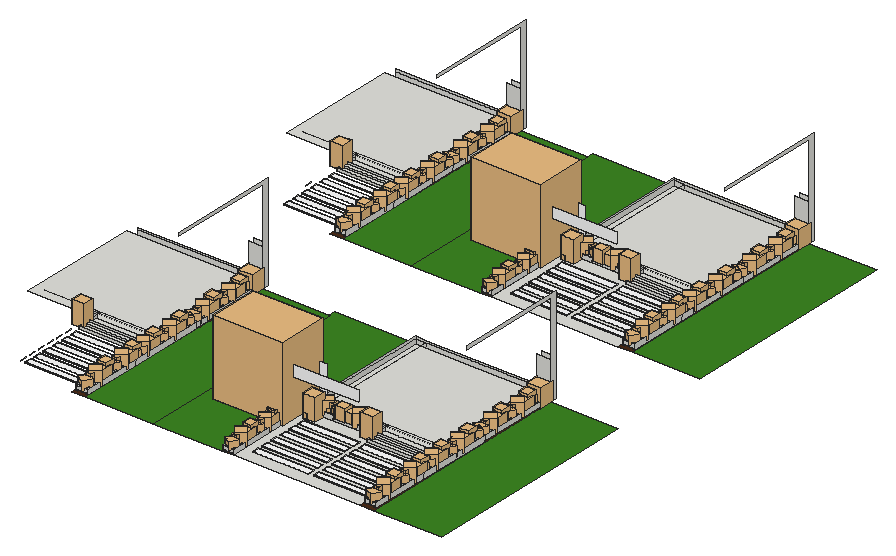
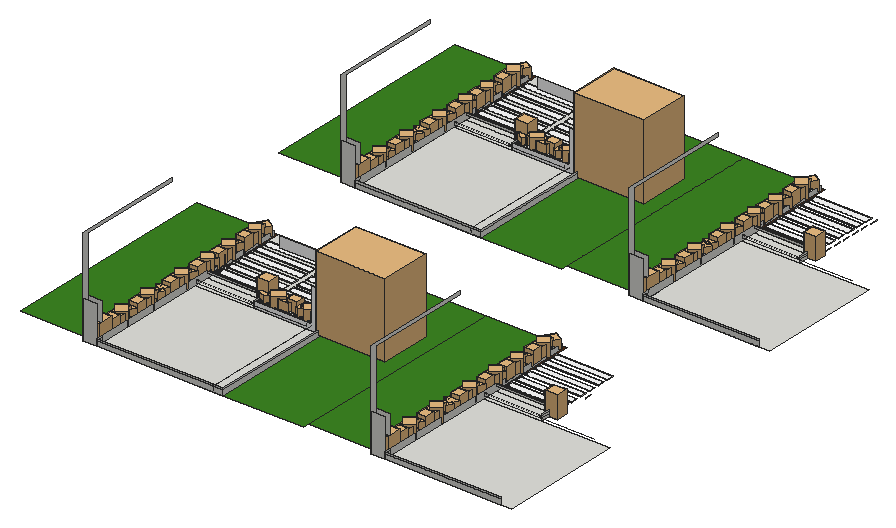
# SketchUp Ruby script. Lengths in inches.
U = 1.inch
M = Sketchup.active_model
def pt(a) = Geom::Point3d.new(a.map { |v| v * U })
def face(e, loops, mat)
  f = e.add_face(loops[0].map { |a| pt(a) })
  loops[1..].each { |l| e.add_face(l.map { |a| pt(a) }).erase! }
  f.material = f.back_material = mat if mat
  f
end
# faces: each face lists its corners as indices into pts; further lists are holes
def faces(e, pts, list, mat = nil) = list.each { |f| face(e, (f[0].is_a?(Array) ? f : [f]).map { |l| l.map { |i| pts[i] } }, mat) }
# xy, xz, yz: faces in a plane at the given z, y or x. An outline is a flat list of corners, or four numbers for a rectangle; further outlines are holes
def ring(l) = l.size == 4 ? [[l[0], l[1]], [l[2], l[1]], [l[2], l[3]], [l[0], l[3]]] : l.each_slice(2).to_a
def flat(e, list, mat, &to3) = list.each { |f| face(e, (f[0].is_a?(Array) ? f : [f]).map { |l| ring(l).map { |u, v| to3.(u, v) } }, mat) }
def xy(e, z, list, mat = nil) = flat(e, list, mat) { |x, y| [x, y, z] }
def xz(e, y, list, mat = nil) = flat(e, list, mat) { |x, z| [x, y, z] }
def yz(e, x, list, mat = nil) = flat(e, list, mat) { |y, z| [x, y, z] }
def lines(e, pts, list) = list.each { |a, b| e.add_line(pt(pts[a]), pt(pts[b])) }
# prism: a flat outline (further loops are holes) pulled along v
def prism(e, loops, v, mat = nil)
  f = face(e, loops, mat); d = Geom::Vector3d.new(v.map { |x| x * U })
  f.pushpull(f.normal.samedirection?(d) ? d.length : -d.length)
end
def box(e, o, s, mat = nil) = prism(e, [[o, [o[0] + s[0], o[1], o[2]], [o[0] + s[0], o[1] + s[1], o[2]], [o[0], o[1] + s[1], o[2]]]], [0, 0, s[2]], mat)
def at(x, y, z, deg = 0) = Geom::Transformation.translation(pt([x, y, z])) * Geom::Transformation.rotation(ORIGIN, Z_AXIS, deg.degrees)
def axes(o, x, y, z) = Geom::Transformation.new([*x, 0, *y, 0, *z, 0, *pt(o).to_a, 1])
def part(name) = M.definitions.add(name)
# library, detail: a bought-in or finely detailed component or shape, given as its bounding box
def library(name, o, s) = part(name).tap { |d| box(d.entities, o, s) }
def detail(e, o, s) = box(e.add_group.entities, o, s)
def put(e, d, t, mat = nil) = e.add_instance(d, t).tap { |i| i.material = mat if mat }
def group(e, t, mat = nil) = e.add_group.tap { |g| g.transformation = t; g.material = mat if mat }.entities
root = M.entities
M.materials.add("Material__1").color = [95, 70, 46]
M.materials.add("[Carrera Marble]").color = [255, 255, 255]
M.materials.add("[Color M00]").color = [255, 255, 255]
M.materials.add("[Color M04]").color = [60, 133, 34]
M.materials.add("[Wood Veneer 01]").color = [76, 44, 23]
c1 = library("plant1",[-367.84,-375.82,-125.45],[750.59,696.16,1346.74])
c2 = part("skp4FF")
put(c2.entities,c1,at(0,0,0))
c3 = library("Areca palm plant",[0,0,0],[49.1,36.6,54.46])
c4 = library("Group\#14",[-84.69,-90.07,-0.36],[176.51,175.13,171.4])
c5 = library("Group20\#1",[-20.81,-17.08,3.79],[39.86,39.43,37.51])
c6 = library("Group\#130",[-7.34,-1.2,0],[38.67,35.81,49.04])
c7 = library("Group38\#2",[14.01,28.44,-23.43],[18.58,18.32,38.89])
c8 = part("Group\#15")
xy(c8.entities,0,[[0,0,6,234.8],[30,0,36,234.8]])
xy(c8.entities,3,[[6,0,30,234.8]])
xy(c8.entities,7,[[6,5,30,229.8]],"Material__1")
xy(c8.entities,15,[[[0,0,36,234.8],[6,5,30,229.8]]])
xz(c8.entities,0,[[0,0,6,0,6,3,30,3,30,0,36,0,36,15,0,15]])
xz(c8.entities,5,[[6,7,30,15]])
xz(c8.entities,229.8,[[6,7,30,15]])
xz(c8.entities,234.8,[[0,0,0,15,36,15,36,0,30,0,30,3,6,3,6,0]])
yz(c8.entities,0,[[0,0,234.8,15]])
yz(c8.entities,6,[[0,0,234.8,3],[5,7,229.8,15]])
yz(c8.entities,30,[[0,0,234.8,3],[5,7,229.8,15]])
yz(c8.entities,36,[[0,0,234.8,15]])
c9 = part("Group\#17")
put(c9.entities,c3,axes([-6.2,56.6,6.08],[0.45017,-0.56191,0],[0.66137,0.52986,0],[0,0,0.72]))
put(c9.entities,c3,axes([-6.2,158.41,6.08],[0.45017,-0.56191,0],[0.66137,0.52986,0],[0,0,0.72]))
put(c9.entities,c4,axes([14.93,44.05,6.05],[-0.04961,-0.08593,0],[0.08593,-0.04961,0],[0,0,0.10522]))
put(c9.entities,c4,axes([14.93,71.3,6.05],[-0.04961,-0.08593,0],[0.08593,-0.04961,0],[0,0,0.10522]))
put(c9.entities,c5,axes([18.97,79.98,4.77],[0,0.85,0],[-0.85,0,0],[0,0,0.85]))
put(c9.entities,c4,axes([14.93,145.87,6.05],[-0.04961,-0.08593,0],[0.08593,-0.04961,0],[0,0,0.10522]))
put(c9.entities,c4,axes([17.19,15.79,6.07],[-0.08133,-0.14087,0],[0.14087,-0.08133,0],[0,0,0.1725]))
put(c9.entities,c4,axes([17.19,223.04,6.07],[-0.08133,-0.14087,0],[0.14087,-0.08133,0],[0,0,0.1725]))
put(c9.entities,c4,axes([17.19,121.23,6.07],[-0.08133,-0.14087,0],[0.14087,-0.08133,0],[0,0,0.1725]))
put(c9.entities,c6,axes([24.9375,191.72,8],[0,0.79,0],[-0.79,0,0],[0,0,0.79]))
put(c9.entities,c6,axes([24.9375,89.91,8],[0,0.79,0],[-0.79,0,0],[0,0,0.79]))
put(c9.entities,c4,axes([14.93,91.37,6.05],[-0.04961,-0.08593,0],[0.08593,-0.04961,0],[0,0,0.10522]))
put(c9.entities,c5,axes([18.97,181.79,4.77],[0,0.85,0],[-0.85,0,0],[0,0,0.85]))
put(c9.entities,c7,axes([-4.1,-1.15,28.17],[0.8848,0,0],[0,0.94674,0],[0,0,0.85826]))
put(c9.entities,c7,axes([-4.1,100.66,28.17],[0.8848,0,0],[0,0.94674,0],[0,0,0.85826]))
put(c9.entities,c8,at(0,0,0))
put(c9.entities,c4,axes([14.93,173.12,6.05],[-0.04961,-0.08593,0],[0.08593,-0.04961,0],[0,0,0.10522]))
put(c9.entities,c4,axes([14.93,193.18,6.05],[-0.04961,-0.08593,0],[0.08593,-0.04961,0],[0,0,0.10522]))
c10 = library("plant (1)",[-35.72,-28.42,0],[66.31,67.39,84.38])
c11 = library("Group\#18",[0,0,0],[68.35,49.34,73.02])
c12 = library("Plant",[0,0,0],[12.59,12.59,14.16])
c13 = part("Group\#16")
put(c13.entities,c3,axes([-6.2,158.41,6.08],[0.45017,-0.56191,0],[0.66137,0.52986,0],[0,0,0.72]))
put(c13.entities,c3,axes([-6.2,56.6,6.08],[0.45017,-0.56191,0],[0.66137,0.52986,0],[0,0,0.72]))
put(c13.entities,c4,axes([14.93,91.37,6.05],[-0.04961,-0.08593,0],[0.08593,-0.04961,0],[0,0,0.10522]))
put(c13.entities,c4,axes([14.93,145.87,6.05],[-0.04961,-0.08593,0],[0.08593,-0.04961,0],[0,0,0.10522]))
put(c13.entities,c4,axes([17.19,223.04,6.07],[-0.08133,-0.14087,0],[0.14087,-0.08133,0],[0,0,0.1725]))
put(c13.entities,c8,at(0,0,0))
put(c13.entities,c4,axes([14.93,193.18,6.05],[-0.04961,-0.08593,0],[0.08593,-0.04961,0],[0,0,0.10522]))
put(c13.entities,c4,axes([17.19,15.79,6.07],[-0.08133,-0.14087,0],[0.14087,-0.08133,0],[0,0,0.1725]))
put(c13.entities,c5,axes([18.97,181.79,4.77],[0,0.85,0],[-0.85,0,0],[0,0,0.85]))
put(c13.entities,c5,axes([18.97,79.98,4.77],[0,0.85,0],[-0.85,0,0],[0,0,0.85]))
put(c13.entities,c7,axes([-4.1,-1.15,28.17],[0.8848,0,0],[0,0.94674,0],[0,0,0.85826]))
put(c13.entities,c7,axes([-4.1,100.66,28.17],[0.8848,0,0],[0,0.94674,0],[0,0,0.85826]))
put(c13.entities,c6,axes([24.9375,89.91,8],[0,0.79,0],[-0.79,0,0],[0,0,0.79]))
put(c13.entities,c4,axes([14.93,173.12,6.05],[-0.04961,-0.08593,0],[0.08593,-0.04961,0],[0,0,0.10522]))
put(c13.entities,c4,axes([14.93,44.05,6.05],[-0.04961,-0.08593,0],[0.08593,-0.04961,0],[0,0,0.10522]))
put(c13.entities,c4,axes([14.93,71.3,6.05],[-0.04961,-0.08593,0],[0.08593,-0.04961,0],[0,0,0.10522]))
put(c13.entities,c6,axes([24.9375,191.72,8],[0,0.79,0],[-0.79,0,0],[0,0,0.79]))
put(c13.entities,c4,axes([17.19,121.23,6.07],[-0.08133,-0.14087,0],[0.14087,-0.08133,0],[0,0,0.1725]))
xy(root,-14.85,[[[2957.51,315.5,3349.13,315.5,3349.13,568.0625,3169.48,568.0625,3169.48,636.6875,2957.51,636.6875,2957.51,593.125,2930.51,593.125,2930.51,586.4375,2957.51,586.4375],[3171.73,497.23,3345.23,518.73],[2983.23,497.23,3156.73,518.73],[3171.73,532.29,3345.23,553.79],[3171.73,462.17,3345.23,483.67],[3171.73,427.11,3345.23,448.61],[3171.73,392.04,3345.23,413.54],[3171.73,356.98,3345.23,378.48],[2983.23,532.29,3156.73,553.79],[2983.23,462.17,3156.73,483.67],[2983.23,427.11,3156.73,448.61],[2983.23,392.04,3156.73,413.54],[2983.23,356.98,3156.73,378.48]],[2930.51,536.1875,2957.51,586.4375],[2276.89,568.0625,2456.54,590.5625],[3169.48,568.0625,3349.13,590.5625],[2276.89,590.5625,2456.54,636.6875],
  [3169.48,590.5625,3349.13,636.6875],[2064.92,636.6875,2456.54,1019],[2957.51,636.6875,3349.13,1019],[2456.54,999.35,2500.29,1019],[3349.13,999.35,3392.88,1019],
  [[2957.51,1314.85,3349.13,1314.85,3349.13,1567.42,3169.48,1567.42,3169.48,1636.04,2957.51,1636.04,2957.51,1592.48,2930.51,1592.48,2930.51,1585.79,2957.51,1585.79],[3171.73,1531.65,3345.23,1553.15],[3171.73,1496.59,3345.23,1518.09],[3171.73,1461.52,3345.23,1483.02],[3171.73,1426.46,3345.23,1447.96],[3171.73,1391.4,3345.23,1412.9],[3171.73,1356.34,3345.23,1377.84],[2983.23,1531.65,3156.73,1553.15],[2983.23,1496.59,3156.73,1518.09],[2983.23,1461.52,3156.73,1483.02],[2983.23,1426.46,3156.73,1447.96],[2983.23,1391.4,3156.73,1412.9],[2983.23,1356.34,3156.73,1377.84]],[2930.51,1535.54,2957.51,1585.79],[2276.89,1567.42,2456.54,1589.92],[3169.48,1567.42,3349.13,1589.92],[2276.89,1589.92,2456.54,1636.04],
  [3169.48,1589.92,3349.13,1636.04],[2064.92,1636.04,2456.54,2018.36],[2957.51,1636.04,3349.13,2018.36],[2456.54,1998.71,2500.29,2018.36],[3349.13,1998.71,3392.88,2018.36]])
xy(root,-14.85,[[2500.29,315.5,2708.22,999.35],[[2708.22,315.5,2930.51,315.5,2930.51,593.125,2957.51,593.125,2957.51,1019,2708.22,1019],[2851.78,562.6,2854.94,565.76,2854.94,562.6]],[3392.88,315.5,3600.8125,999.35],[2851.78,562.6,2854.94,562.6,2854.94,565.76],[2500.29,1314.85,2708.22,1998.71],
  [[2708.22,1314.85,2930.51,1314.85,2930.51,1592.48,2957.51,1592.48,2957.51,2018.36,2708.22,2018.36],[2851.78,1561.96,2854.94,1565.12,2854.94,1561.96]],[3392.88,1314.85,3600.8125,1998.71],[2851.78,1561.96,2854.94,1561.96,2854.94,1565.12]],"[Color M04]")
xy(root,-14.85,[[2456.54,315.5,2500.29,999.35],[2930.51,315.5,2957.51,536.1875],[3349.13,315.5,3392.88,999.35],[2456.54,1314.85,2500.29,1998.71],[2930.51,1314.85,2957.51,1535.54],
  [3349.13,1314.85,3392.88,1998.71]],"[Wood Veneer 01]")
xy(root,-13.54,[[2279.14,356.98,2452.64,378.48],[2983.23,356.98,3156.73,378.48],[3171.73,356.98,3345.23,378.48],[2279.14,392.04,2452.64,413.54],[2983.23,392.04,3156.73,413.54],
  [3171.73,392.04,3345.23,413.54],[2279.14,427.11,2452.64,448.61],[2983.23,427.11,3156.73,448.61],[3171.73,427.11,3345.23,448.61],[2279.14,462.17,2452.64,483.67],
  [2983.23,462.17,3156.73,483.67],[3171.73,462.17,3345.23,483.67],[2279.14,497.23,2452.64,518.73],[2983.23,497.23,3156.73,518.73],[3171.73,497.23,3345.23,518.73],
  [2279.14,532.29,2452.64,553.79],[2983.23,532.29,3156.73,553.79],[3171.73,532.29,3345.23,553.79],[2279.14,1356.34,2452.64,1377.84],[2983.23,1356.34,3156.73,1377.84],
  [3171.73,1356.34,3345.23,1377.84],[2279.14,1391.4,2452.64,1412.9],[2983.23,1391.4,3156.73,1412.9],[3171.73,1391.4,3345.23,1412.9],[2279.14,1426.46,2452.64,1447.96],
  [2983.23,1426.46,3156.73,1447.96],[3171.73,1426.46,3345.23,1447.96],[2279.14,1461.52,2452.64,1483.02],[2983.23,1461.52,3156.73,1483.02],[3171.73,1461.52,3345.23,1483.02],
  [2279.14,1496.59,2452.64,1518.09],[2983.23,1496.59,3156.73,1518.09],[3171.73,1496.59,3345.23,1518.09],[2279.14,1531.65,2452.64,1553.15],[2983.23,1531.65,3156.73,1553.15],
  [3171.73,1531.65,3345.23,1553.15]],"[Carrera Marble]")
xy(root,-6.43,[[2276.89,568.0625,2456.54,579.9375],[3169.48,568.0625,3349.13,579.9375],[2276.89,1567.42,2456.54,1579.29],[3169.48,1567.42,3349.13,1579.29]])
xy(root,-0.05,[[2276.89,579.9375,2456.54,590.5625],[3169.48,579.9375,3349.13,590.5625],[2276.89,1579.29,2456.54,1589.92],[3169.48,1579.29,3349.13,1589.92]])
xz(root,356.98,[[2279.14,-14.85,2452.64,-13.54],[2983.23,-14.85,3156.73,-13.54],[3171.73,-14.85,3345.23,-13.54]])
xz(root,378.48,[[2279.14,-14.85,2452.64,-13.54],[2983.23,-14.85,3156.73,-13.54],[3171.73,-14.85,3345.23,-13.54]])
xz(root,392.04,[[2279.14,-14.85,2452.64,-13.54],[2983.23,-14.85,3156.73,-13.54],[3171.73,-14.85,3345.23,-13.54]])
xz(root,413.54,[[2279.14,-14.85,2452.64,-13.54],[2983.23,-14.85,3156.73,-13.54],[3171.73,-14.85,3345.23,-13.54]])
xz(root,427.11,[[2279.14,-14.85,2452.64,-13.54],[2983.23,-14.85,3156.73,-13.54],[3171.73,-14.85,3345.23,-13.54]])
xz(root,448.61,[[2279.14,-14.85,2452.64,-13.54],[2983.23,-14.85,3156.73,-13.54],[3171.73,-14.85,3345.23,-13.54]])
xz(root,462.17,[[2279.14,-14.85,2452.64,-13.54],[2983.23,-14.85,3156.73,-13.54],[3171.73,-14.85,3345.23,-13.54]])
xz(root,483.67,[[2279.14,-14.85,2452.64,-13.54],[2983.23,-14.85,3156.73,-13.54],[3171.73,-14.85,3345.23,-13.54]])
xz(root,497.23,[[2279.14,-14.85,2452.64,-13.54],[2983.23,-14.85,3156.73,-13.54],[3171.73,-14.85,3345.23,-13.54]])
xz(root,518.73,[[2279.14,-14.85,2452.64,-13.54],[2983.23,-14.85,3156.73,-13.54],[3171.73,-14.85,3345.23,-13.54]])
xz(root,532.29,[[2279.14,-14.85,2452.64,-13.54],[2983.23,-14.85,3156.73,-13.54],[3171.73,-14.85,3345.23,-13.54]])
xz(root,536.1875,[[2930.51,-14.85,2957.51,-14.85,2957.51,109.625,3169.48,109.625,3169.48,142.875,2930.51,142.875]],"[Color M00]")
xz(root,553.79,[[2279.14,-14.85,2452.64,-13.54],[2983.23,-14.85,3156.73,-13.54],[3171.73,-14.85,3345.23,-13.54]])
xz(root,568.0625,[[2276.89,-14.85,2456.54,-6.43],[3169.48,-14.85,3349.13,-6.43]])
xz(root,579.9375,[[2276.89,-6.43,2456.54,-0.05],[3169.48,-6.43,3349.13,-0.05]])
xz(root,586.4375,[[2930.51,-14.85,2957.51,109.5]])
xz(root,590.5625,[[2276.89,-0.05,2456.54,6],[3169.48,-0.05,3349.13,6]])
xz(root,636.6875,[[2276.89,-0.05,2456.54,0],[3169.48,-0.05,3349.13,0]])
xz(root,636.6875,[[2957.51,-14.85,3169.48,-14.85,3169.48,6,2989.82,6,2989.82,109.5,2957.51,109.5]],"[Color M00]")
xz(root,999.35,[[2456.54,-14.85,2500.29,102.625],[3349.13,-14.85,3392.88,102.625]])
xz(root,1019,[[2097.23,-14.85,2456.54,0],[2456.54,-14.85,2500.29,102.625],[2957.51,-14.85,2989.82,0],[2989.82,-14.85,3349.13,0],[3349.13,-14.85,3392.88,102.625],
  [2097.23,0,2456.54,6],[2957.51,0,2989.82,6],[2989.82,0,3349.13,6]])
xz(root,1356.34,[[2279.14,-14.85,2452.64,-13.54],[2983.23,-14.85,3156.73,-13.54],[3171.73,-14.85,3345.23,-13.54]])
xz(root,1377.84,[[2279.14,-14.85,2452.64,-13.54],[2983.23,-14.85,3156.73,-13.54],[3171.73,-14.85,3345.23,-13.54]])
xz(root,1391.4,[[2279.14,-14.85,2452.64,-13.54],[2983.23,-14.85,3156.73,-13.54],[3171.73,-14.85,3345.23,-13.54]])
xz(root,1412.9,[[2279.14,-14.85,2452.64,-13.54],[2983.23,-14.85,3156.73,-13.54],[3171.73,-14.85,3345.23,-13.54]])
xz(root,1426.46,[[2279.14,-14.85,2452.64,-13.54],[2983.23,-14.85,3156.73,-13.54],[3171.73,-14.85,3345.23,-13.54]])
xz(root,1447.96,[[2279.14,-14.85,2452.64,-13.54],[2983.23,-14.85,3156.73,-13.54],[3171.73,-14.85,3345.23,-13.54]])
xz(root,1461.52,[[2279.14,-14.85,2452.64,-13.54],[2983.23,-14.85,3156.73,-13.54],[3171.73,-14.85,3345.23,-13.54]])
xz(root,1483.02,[[2279.14,-14.85,2452.64,-13.54],[2983.23,-14.85,3156.73,-13.54],[3171.73,-14.85,3345.23,-13.54]])
xz(root,1496.59,[[2279.14,-14.85,2452.64,-13.54],[2983.23,-14.85,3156.73,-13.54],[3171.73,-14.85,3345.23,-13.54]])
xz(root,1518.09,[[2279.14,-14.85,2452.64,-13.54],[2983.23,-14.85,3156.73,-13.54],[3171.73,-14.85,3345.23,-13.54]])
xz(root,1531.65,[[2279.14,-14.85,2452.64,-13.54],[2983.23,-14.85,3156.73,-13.54],[3171.73,-14.85,3345.23,-13.54]])
xz(root,1535.54,[[2930.51,-14.85,2957.51,-14.85,2957.51,109.625,3169.48,109.625,3169.48,142.875,2930.51,142.875]],"[Color M00]")
xz(root,1553.15,[[2279.14,-14.85,2452.64,-13.54],[2983.23,-14.85,3156.73,-13.54],[3171.73,-14.85,3345.23,-13.54]])
xz(root,1567.42,[[2276.89,-14.85,2456.54,-6.43],[3169.48,-14.85,3349.13,-6.43]])
xz(root,1579.29,[[2276.89,-6.43,2456.54,-0.05],[3169.48,-6.43,3349.13,-0.05]])
xz(root,1585.79,[[2930.51,-14.85,2957.51,109.5]])
xz(root,1589.92,[[2276.89,-0.05,2456.54,6],[3169.48,-0.05,3349.13,6]])
xz(root,1636.04,[[2276.89,-0.05,2456.54,0],[3169.48,-0.05,3349.13,0]])
xz(root,1636.04,[[2957.51,-14.85,3169.48,-14.85,3169.48,6,2989.82,6,2989.82,109.5,2957.51,109.5]],"[Color M00]")
xz(root,1998.71,[[2456.54,-14.85,2500.29,102.625],[3349.13,-14.85,3392.88,102.625]])
xz(root,2018.36,[[2097.23,-14.85,2456.54,0],[2456.54,-14.85,2500.29,102.625],[2957.51,-14.85,2989.82,0],[2989.82,-14.85,3349.13,0],[3349.13,-14.85,3392.88,102.625],
  [2097.23,0,2456.54,6],[2957.51,0,2989.82,6],[2989.82,0,3349.13,6]])
yz(root,2264.14,[[356.98,-14.85,378.48,-13.54],[392.04,-14.85,413.54,-13.54],[427.11,-14.85,448.61,-13.54],[462.17,-14.85,483.67,-13.54],[497.23,-14.85,518.73,-13.54],
  [532.29,-14.85,553.79,-13.54],[1461.52,-14.85,1483.02,-13.54]])
yz(root,2276.89,[[568.0625,-14.85,590.5625,-6.43],[590.5625,-14.85,636.6875,-6.43],[1567.42,-14.85,1589.92,-6.43],[1589.92,-14.85,1636.04,-6.43],[579.9375,-6.43,590.5625,-0.05],
  [590.5625,-6.43,636.6875,-0.05],[1579.29,-6.43,1589.92,-0.05],[1589.92,-6.43,1636.04,-0.05],[590.5625,-0.05,636.6875,6],[1589.92,-0.05,1636.04,6]])
yz(root,2279.14,[[356.98,-14.85,378.48,-13.54],[392.04,-14.85,413.54,-13.54],[427.11,-14.85,448.61,-13.54],[462.17,-14.85,483.67,-13.54],[497.23,-14.85,518.73,-13.54],
  [532.29,-14.85,553.79,-13.54],[1356.34,-14.85,1377.84,-13.54],[1391.4,-14.85,1412.9,-13.54],[1426.46,-14.85,1447.96,-13.54],[1461.52,-14.85,1483.02,-13.54],
  [1496.59,-14.85,1518.09,-13.54],[1531.65,-14.85,1553.15,-13.54]])
yz(root,2452.64,[[356.98,-14.85,378.48,-13.54],[392.04,-14.85,413.54,-13.54],[427.11,-14.85,448.61,-13.54],[462.17,-14.85,483.67,-13.54],[497.23,-14.85,518.73,-13.54],
  [532.29,-14.85,553.79,-13.54],[1356.34,-14.85,1377.84,-13.54],[1391.4,-14.85,1412.9,-13.54],[1426.46,-14.85,1447.96,-13.54],[1461.52,-14.85,1483.02,-13.54],
  [1496.59,-14.85,1518.09,-13.54],[1531.65,-14.85,1553.15,-13.54]])
yz(root,2456.54,[[568.0625,-14.85,999.35,-14.85,999.35,6,590.5625,6,590.5625,-0.05,579.9375,-0.05,579.9375,-6.43,568.0625,-6.43],[999.35,-14.85,1019,0],[1567.42,-14.85,1998.71,-14.85,1998.71,6,1589.92,6,1589.92,-0.05,1579.29,-0.05,1579.29,-6.43,1567.42,-6.43],[1998.71,-14.85,2018.36,0],[999.35,0,1019,6],
  [1998.71,0,2018.36,6]])
yz(root,2500.29,[[999.35,-14.85,1019,-14.85,1019,283.9375,674.36,283.9375,674.36,274.0625,999.35,274.0625],[1998.71,-14.85,2018.36,-14.85,2018.36,283.9375,1673.72,283.9375,1673.72,274.0625,1998.71,274.0625]])
yz(root,2930.51,[[536.1875,-14.85,536.1875,142.875,636.6875,142.875,636.6875,109.5,586.4375,109.5,586.4375,-14.85],[1535.54,-14.85,1535.54,142.875,1636.04,142.875,1636.04,109.5,1585.79,109.5,1585.79,-14.85]])
yz(root,2957.51,[[636.6875,-14.85,1019,0],[1636.04,-14.85,2018.36,0],[636.6875,0,1019,6],[1636.04,0,2018.36,6]])
yz(root,2957.51,[[536.1875,-14.85,586.4375,-14.85,586.4375,109.5,636.6875,109.5,636.6875,109.625,536.1875,109.625],[1535.54,-14.85,1585.79,-14.85,1585.79,109.5,1636.04,109.5,1636.04,109.625,1535.54,109.625]],"[Wood Veneer 01]")
yz(root,2983.23,[[356.98,-14.85,378.48,-13.54],[392.04,-14.85,413.54,-13.54],[427.11,-14.85,448.61,-13.54],[462.17,-14.85,483.67,-13.54],[497.23,-14.85,518.73,-13.54],
  [532.29,-14.85,553.79,-13.54],[1356.34,-14.85,1377.84,-13.54],[1391.4,-14.85,1412.9,-13.54],[1426.46,-14.85,1447.96,-13.54],[1461.52,-14.85,1483.02,-13.54],
  [1496.59,-14.85,1518.09,-13.54],[1531.65,-14.85,1553.15,-13.54]])
yz(root,3156.73,[[356.98,-14.85,378.48,-13.54],[392.04,-14.85,413.54,-13.54],[427.11,-14.85,448.61,-13.54],[462.17,-14.85,483.67,-13.54],[497.23,-14.85,518.73,-13.54],
  [532.29,-14.85,553.79,-13.54],[1356.34,-14.85,1377.84,-13.54],[1391.4,-14.85,1412.9,-13.54],[1426.46,-14.85,1447.96,-13.54],[1461.52,-14.85,1483.02,-13.54],
  [1496.59,-14.85,1518.09,-13.54],[1531.65,-14.85,1553.15,-13.54]])
yz(root,3169.48,[[568.0625,-14.85,590.5625,-6.43],[590.5625,-14.85,636.6875,-6.43],[1567.42,-14.85,1589.92,-6.43],[1589.92,-14.85,1636.04,-6.43],[579.9375,-6.43,590.5625,-0.05],
  [590.5625,-6.43,636.6875,-0.05],[1579.29,-6.43,1589.92,-0.05],[1589.92,-6.43,1636.04,-0.05],[590.5625,-0.05,636.6875,6],[1589.92,-0.05,1636.04,6]])
yz(root,3171.73,[[356.98,-14.85,378.48,-13.54],[392.04,-14.85,413.54,-13.54],[427.11,-14.85,448.61,-13.54],[462.17,-14.85,483.67,-13.54],[497.23,-14.85,518.73,-13.54],
  [532.29,-14.85,553.79,-13.54],[1356.34,-14.85,1377.84,-13.54],[1391.4,-14.85,1412.9,-13.54],[1426.46,-14.85,1447.96,-13.54],[1461.52,-14.85,1483.02,-13.54],
  [1496.59,-14.85,1518.09,-13.54],[1531.65,-14.85,1553.15,-13.54]])
yz(root,3345.23,[[356.98,-14.85,378.48,-13.54],[392.04,-14.85,413.54,-13.54],[427.11,-14.85,448.61,-13.54],[462.17,-14.85,483.67,-13.54],[497.23,-14.85,518.73,-13.54],
  [532.29,-14.85,553.79,-13.54],[1356.34,-14.85,1377.84,-13.54],[1391.4,-14.85,1412.9,-13.54],[1426.46,-14.85,1447.96,-13.54],[1461.52,-14.85,1483.02,-13.54],
  [1496.59,-14.85,1518.09,-13.54],[1531.65,-14.85,1553.15,-13.54]])
yz(root,3349.13,[[568.0625,-14.85,999.35,-14.85,999.35,6,590.5625,6,590.5625,-0.05,579.9375,-0.05,579.9375,-6.43,568.0625,-6.43],[999.35,-14.85,1019,0],[1567.42,-14.85,1998.71,-14.85,1998.71,6,1589.92,6,1589.92,-0.05,1579.29,-0.05,1579.29,-6.43,1567.42,-6.43],[1998.71,-14.85,2018.36,0],[999.35,0,1019,6],
  [1998.71,0,2018.36,6]])
yz(root,3392.88,[[999.35,-14.85,1019,-14.85,1019,283.9375,674.36,283.9375,674.36,274.0625,999.35,274.0625],[1998.71,-14.85,2018.36,-14.85,2018.36,283.9375,1673.72,283.9375,1673.72,274.0625,1998.71,274.0625]])
p = [[2447.32,645.91,0],[2447.32,645.91,6],[2447.32,645.91,-1.6875],[2106.46,645.91,0],[2999.05,645.91,0],[3339.91,645.91,0],
  [3339.91,645.91,6],[2999.05,645.91,6],[2999.05,645.91,-1.6875],[3339.91,645.91,-1.6875],[2989.82,1019,0],[2989.82,636.6875,0],
  [2106.46,1645.27,0],[2447.32,1645.27,0],[2447.32,1645.27,6],[2999.05,1645.27,0],[2999.05,1645.27,-1.6875],[2447.32,1645.27,-1.6875],
  [2989.82,2018.36,0],[2989.82,1636.04,0],[3339.91,1645.27,0],[3339.91,1645.27,-1.6875],[3339.91,1645.27,6],[2999.05,1645.27,6]]
lines(root,p,[[0,1],[0,2],[3,0],[4,5],[5,6],[4,7],[4,8],[5,9],[10,11],[12,13],[13,14],[15,16],
  [13,17],[18,19],[20,21],[20,22],[15,23],[15,20]])
put(root,c2,axes([2268.84,1592.3,-5.92],[0.05049,0,0],[0,0.05049,0],[0,0,0.05049]))
put(root,c2,axes([2268.84,592.95,-5.92],[0.05049,0,0],[0,0.05049,0],[0,0,0.05049]))
put(root,c9,at(2460.18,1511.48,-14.85))
put(root,c9,at(2460.18,1742.1,-14.85))
put(root,c9,at(2460.18,1327.53,-14.85))
put(root,c9,at(2460.18,742.75,-14.85))
put(root,c9,at(2460.18,512.125,-14.85))
put(root,c9,at(2460.18,328.17,-14.85))
put(root,c10,axes([2480.48,1978.05,-14.85],[0.67,0,0],[0,0.67,0],[0,0,0.67]))
put(root,c10,axes([2480.48,978.7,-14.85],[0.67,0,0],[0,0.67,0],[0,0,0.67]))
put(root,c11,axes([2749.84,1494.25,-9.3125],[3.16,0,0],[0,3.16,0],[0,0,3.16]))
put(root,c11,axes([2749.84,494.9,-9.3125],[3.16,0,0],[0,3.16,0],[0,0,3.16]))
put(root,c9,axes([2922.71,1318.59,-14.85],[0.92,0,0],[0,0.92,0],[0,0,0.92]))
put(root,c9,axes([2922.71,319.23,-14.85],[0.92,0,0],[0,0.92,0],[0,0,0.92]))
put(root,c12,at(2972.82,1563.1,-13.54))
put(root,c12,at(2972.82,563.75,-13.54))
put(root,c2,axes([2992.09,1582.8,-7.21],[0.05049,0,0],[0,0.05049,0],[0,0,0.05049]))
put(root,c2,axes([2992.09,583.44,-7.21],[0.05049,0,0],[0,0.05049,0],[0,0,0.05049]))
put(root,c13,at(3165.42,1592.3,-10.64,90))
put(root,c13,at(3165.42,592.95,-10.64,90))
put(root,c2,axes([3161.43,1592.3,-5.92],[0.05049,0,0],[0,0.05049,0],[0,0,0.05049]))
put(root,c2,axes([3161.43,592.95,-5.92],[0.05049,0,0],[0,0.05049,0],[0,0,0.05049]))
put(root,c9,at(3352.77,1511.48,-14.85))
put(root,c9,at(3352.77,1742.1,-14.85))
put(root,c9,at(3352.77,512.125,-14.85))
put(root,c9,at(3352.77,742.75,-14.85))
put(root,c9,at(3352.77,1327.53,-14.85))
put(root,c9,at(3352.77,328.17,-14.85))
put(root,c10,axes([3373.07,1978.05,-14.85],[0.67,0,0],[0,0.67,0],[0,0,0.67]))
put(root,c10,axes([3373.07,978.7,-14.85],[0.67,0,0],[0,0.67,0],[0,0,0.67]))
